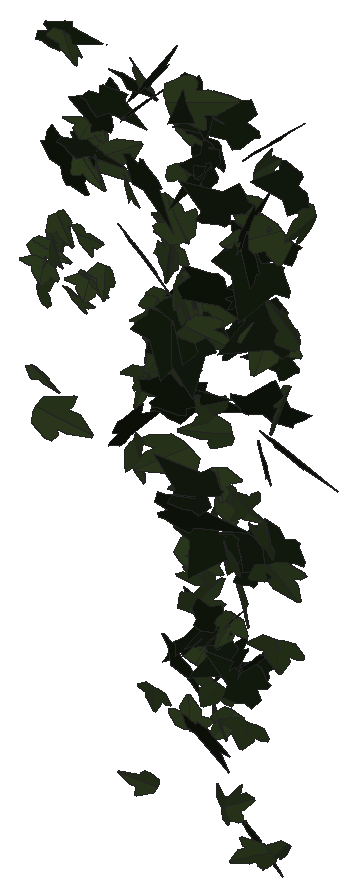
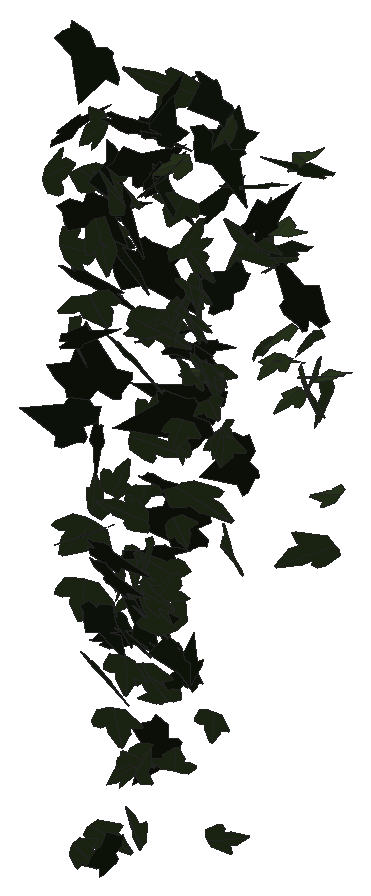
# SketchUp Ruby script. Lengths in inches.
U = 1.inch
M = Sketchup.active_model
def pt(a) = Geom::Point3d.new(a.map { |v| v * U })
def face(e, loops, mat)
  f = e.add_face(loops[0].map { |a| pt(a) })
  loops[1..].each { |l| e.add_face(l.map { |a| pt(a) }).erase! }
  f.material = f.back_material = mat if mat
  f
end
# faces: each face lists its corners as indices into pts; further lists are holes
def faces(e, pts, list, mat = nil) = list.each { |f| face(e, (f[0].is_a?(Array) ? f : [f]).map { |l| l.map { |i| pts[i] } }, mat) }
# xy, xz, yz: faces in a plane at the given z, y or x. An outline is a flat list of corners, or four numbers for a rectangle; further outlines are holes
def ring(l) = l.size == 4 ? [[l[0], l[1]], [l[2], l[1]], [l[2], l[3]], [l[0], l[3]]] : l.each_slice(2).to_a
def flat(e, list, mat, &to3) = list.each { |f| face(e, (f[0].is_a?(Array) ? f : [f]).map { |l| ring(l).map { |u, v| to3.(u, v) } }, mat) }
def xy(e, z, list, mat = nil) = flat(e, list, mat) { |x, y| [x, y, z] }
def xz(e, y, list, mat = nil) = flat(e, list, mat) { |x, z| [x, y, z] }
def yz(e, x, list, mat = nil) = flat(e, list, mat) { |y, z| [x, y, z] }
def lines(e, pts, list) = list.each { |a, b| e.add_line(pt(pts[a]), pt(pts[b])) }
# prism: a flat outline (further loops are holes) pulled along v
def prism(e, loops, v, mat = nil)
  f = face(e, loops, mat); d = Geom::Vector3d.new(v.map { |x| x * U })
  f.pushpull(f.normal.samedirection?(d) ? d.length : -d.length)
end
def box(e, o, s, mat = nil) = prism(e, [[o, [o[0] + s[0], o[1], o[2]], [o[0] + s[0], o[1] + s[1], o[2]], [o[0], o[1] + s[1], o[2]]]], [0, 0, s[2]], mat)
def at(x, y, z, deg = 0) = Geom::Transformation.translation(pt([x, y, z])) * Geom::Transformation.rotation(ORIGIN, Z_AXIS, deg.degrees)
def axes(o, x, y, z) = Geom::Transformation.new([*x, 0, *y, 0, *z, 0, *pt(o).to_a, 1])
def part(name) = M.definitions.add(name)
# library, detail: a bought-in or finely detailed component or shape, given as its bounding box
def library(name, o, s) = part(name).tap { |d| box(d.entities, o, s) }
def detail(e, o, s) = box(e.add_group.entities, o, s)
def put(e, d, t, mat = nil) = e.add_instance(d, t).tap { |i| i.material = mat if mat }
def group(e, t, mat = nil) = e.add_group.tap { |g| g.transformation = t; g.material = mat if mat }.entities
root = M.entities
M.materials.add("1026 AP 7946 SUNNY SIDE UP").color = [254, 231, 186]
M.materials.add("efeu1").color = [18, 25, 13]
M.materials.add("efeu2").color = [43, 57, 29]
c1 = part("ivyleaf_10")
p = [[0,0.5,-0.03],[-0.0625,2.02,-0.43],[-0.19,2.01,-0.46],[-0.54,1.05,-0.29],[-0.52,0.625,-0.18],[-0.83,0.76,-0.28],
  [-1.16,0.64,-0.33],[-1.15,0.33,-0.24],[-0.77,-0.39,0.02],[-0.3,-0.51,0.16],[0.04,-0.48,0.23],[-0.02,2.01,-0.4375],
  [-0.06,2.01,-0.43],[0.04,-0.49,0.23],[0.67,-0.49,0.14],[1.38,0.36,-0.2],[1.375,0.51,-0.24],[0.81,0.65,-0.19],
  [0.62,0.59,-0.15],[0.6,1.09,-0.28],[0.5,1.23,-0.31]]
faces(c1.entities,p,[[0,1,2,3,4,5,6,7,8,9,10],[11,12,0,13,14,15,16,17,18,19,20]],"efeu2")
c2 = part("ivyleaf_9")
p = [[1.54,2.16,1.25],[1.36,2.04,1.19],[-0.21,0.99,0.68],[-0.71,1.11,0.82],[-0.85,0.86,0.67],[-0.8,0.17,0.21],
  [-0.9,-0.01,0.1],[-0.67,-0.16,-0.02],[-0.08,-0.08,-0.05],[-0.03,-0.6,-0.4],[0.65,-0.88,-0.66],[0.83,-0.6,-0.49],
  [1.29,-0.42,-0.43],[1.8125,-0.07,-0.26],[1.21,0.44,0.15]]
faces(c2.entities,p,[[0,1,2,3,4,5,6,7,8,9,10,11,12,13,14]],"efeu1")
put(root,c1,axes([138.98,210.22,263.24],[-0.26832,-0.09266,0.10652],[0.15209,-0.19714,-0.01861],[0.15749,0.03251,0.19947]),"1026 AP 7946 SUNNY SIDE UP")
put(root,c1,axes([141.6,210.05,255.69],[-0.31273,0.03362,0.02954],[-0.04908,-0.01456,-0.20692],[-0.0489,-0.20039,0.01878]),"1026 AP 7946 SUNNY SIDE UP")
put(root,c2,axes([143.76,210.15,256.46],[-0.25605,-0.21365,-0.05442],[-0.05292,-0.03924,0.27649],[-0.34152,0.16625,-0.00204]),"1026 AP 7946 SUNNY SIDE UP")
put(root,c2,axes([142,210.32,256.35],[0.31816,-0.22092,-0.16843],[0.20052,-0.10262,0.30721],[-0.3815,-0.23818,0.02101]),"1026 AP 7946 SUNNY SIDE UP")
put(root,c2,axes([143.74,210.33,264.84],[-0.29155,-0.31885,0.04974],[0.01185,-0.06203,-0.37839],[0.50737,-0.18177,0.03742]),"1026 AP 7946 SUNNY SIDE UP")
put(root,c2,axes([141.14,210.23,265.92],[0.26357,-0.32189,0.03584],[0.00376,-0.03999,-0.37373],[0.50938,0.16685,-0.01578]),"1026 AP 7946 SUNNY SIDE UP")
put(root,c1,axes([139.97,210.27,263.22],[-0.30788,-0.07706,0.05458],[0.11552,-0.20293,-0.02532],[0.0916,-0.00305,0.2154]),"1026 AP 7946 SUNNY SIDE UP")
put(root,c1,axes([143.17,210.25,257.56],[0.14453,0.17083,-0.16949],[-0.10294,-0.1524,-0.20041],[-0.35954,0.1123,-0.01076]),"1026 AP 7946 SUNNY SIDE UP")
put(root,c2,axes([142.03,210.28,262.86],[-0.30127,-0.16523,-0.24528],[0.39598,0.04422,-0.24108],[0.22307,-0.30166,0.09668]),"1026 AP 7946 SUNNY SIDE UP")
put(root,c2,axes([143.08,210.27,265.71],[0.06562,0.03036,0.30626],[-0.45026,-0.08115,0.0495],[0.1334,-0.28884,0.01644]),"1026 AP 7946 SUNNY SIDE UP")
put(root,c1,axes([142.92,210.16,256.16],[-0.34394,-0.02236,0.12398],[-0.18185,-0.04373,-0.22494],[0.06363,-0.24586,0.02724]),"1026 AP 7946 SUNNY SIDE UP")
put(root,c2,axes([141.7,210.07,261.63],[0.17769,0.01894,0.30716],[0.4696,-0.00543,-0.11633],[-0.00256,0.31871,-0.01836]),"1026 AP 7946 SUNNY SIDE UP")
put(root,c2,axes([140.98,209.88,260.74],[0.12516,0.14997,0.31618],[0.26676,0.25516,-0.17277],[-0.46482,0.18682,-0.01401]),"1026 AP 7946 SUNNY SIDE UP")
put(root,c2,axes([143.1875,210.25,256.81],[-0.40171,0.02984,0.02023],[-0.03496,-0.02339,-0.26379],[-0.04378,-0.25515,0.02502]),"1026 AP 7946 SUNNY SIDE UP")
put(root,c1,axes([143.41,209.97,254.0625],[-0.00784,0.02709,0.27849],[-0.07168,0.26631,-0.02682],[-0.4209,-0.04585,-0.00062]),"1026 AP 7946 SUNNY SIDE UP")
put(root,c2,axes([140.92,210.36,264.24],[0.23132,-0.24892,0.20326],[0.14646,-0.1757,-0.29879],[0.47893,0.17395,-0.0068]),"1026 AP 7946 SUNNY SIDE UP")
put(root,c2,axes([141.78,210.35,262.9],[-0.2621,-0.26595,-0.02368],[0.04161,0.00871,-0.32278],[0.41747,-0.16784,0.01731]),"1026 AP 7946 SUNNY SIDE UP")
put(root,c2,axes([143.38,210.27,257.04],[-0.29867,0.12568,-0.13501],[0.15186,-0.09188,-0.23425],[-0.24272,-0.21213,0.01957]),"1026 AP 7946 SUNNY SIDE UP")
put(root,c1,axes([138.79,210.25,261.03],[0.00803,-0.18886,0.07584],[0.30325,-0.0189,-0.06294],[0.10008,0.07244,0.18463]),"1026 AP 7946 SUNNY SIDE UP")
put(root,c2,axes([142.97,210.25,257.34],[-0.35126,0.10724,-0.02573],[0.02114,-0.03088,-0.25446],[-0.17206,-0.22272,0.02126]),"1026 AP 7946 SUNNY SIDE UP")
put(root,c1,axes([140.24,210.36,263.46],[-0.10201,-0.17563,0.12827],[0.1628,-0.14031,-0.14796],[0.29784,0.01654,0.12481]),"1026 AP 7946 SUNNY SIDE UP")
put(root,c2,axes([143.01,210.24,264.17],[0.03459,0.13881,-0.34969],[-0.43407,-0.21872,-0.1116],[-0.38135,0.26154,0.0953]),"1026 AP 7946 SUNNY SIDE UP")
put(root,c2,axes([144.2,209.96,267.58],[0.12837,0.33147,0.16836],[0.02917,0.16155,-0.35021],[-0.57907,0.08162,0.01968]),"1026 AP 7946 SUNNY SIDE UP")
put(root,c2,axes([142.58,210.24,259.89],[-0.38041,-0.09691,-0.142],[-0.21271,-0.03045,0.26755],[-0.15676,0.27649,-0.01847]),"1026 AP 7946 SUNNY SIDE UP")
put(root,c2,axes([143.59,210.14,265.2],[0.09755,-0.04066,-0.38485],[-0.58547,0.04263,-0.06827],[0.07692,0.37605,-0.03162]),"1026 AP 7946 SUNNY SIDE UP")
put(root,c1,axes([141.28,210.32,253.6],[-0.08349,-0.02972,-0.20093],[-0.29572,-0.05283,0.06078],[-0.09287,0.19494,-0.01291]),"1026 AP 7946 SUNNY SIDE UP")
put(root,c1,axes([141.64,210.3,262.55],[0.40251,-0.21261,-0.06265],[-0.09805,0.01793,-0.34168],[0.33307,0.26222,-0.02488]),"1026 AP 7946 SUNNY SIDE UP")
put(root,c2,axes([142.72,210.22,257.01],[0.09106,0.26368,0.08717],[-0.04006,-0.07947,0.27754],[0.43287,-0.06282,0.00735]),"1026 AP 7946 SUNNY SIDE UP")
put(root,c1,axes([141.12,210.36,261.54],[0.07408,0.15737,-0.12689],[-0.05346,-0.11932,-0.16992],[-0.31053,0.05809,-0.00102]),"1026 AP 7946 SUNNY SIDE UP")
put(root,c2,axes([141.85,210.21,259.33],[0.33666,0.01357,0.26927],[0.41,-0.03918,-0.21823],[0.03426,0.33554,-0.03438]),"1026 AP 7946 SUNNY SIDE UP")
put(root,c1,axes([142.09,210.1875,267.62],[0.16546,-0.01515,-0.3647],[0.54382,0.08429,0.10271],[0.12054,-0.35949,0.03723]),"1026 AP 7946 SUNNY SIDE UP")
put(root,c1,axes([144.16,210.3,257.4],[-0.42519,-0.08595,0.00603],[0.00354,-0.02791,-0.29112],[0.13547,-0.26904,0.02653]),"1026 AP 7946 SUNNY SIDE UP")
put(root,c2,axes([143.83,210.27,257.08],[-0.10898,0.24451,-0.10809],[0.03027,-0.10497,-0.26226],[-0.41815,-0.07132,0.00919]),"1026 AP 7946 SUNNY SIDE UP")
put(root,c2,axes([142.18,210.625,267.55],[0.11944,-0.19514,-0.32586],[0.2779,-0.26377,0.21056],[-0.51241,-0.18854,0.03824]),"1026 AP 7946 SUNNY SIDE UP")
put(root,c2,axes([142.77,210.25,257.32],[0.00556,0.01588,0.24924],[-0.23403,0.19104,-0.00957],[-0.30078,-0.14835,0.01205]),"1026 AP 7946 SUNNY SIDE UP")
put(root,c2,axes([143.69,210.23,264.46],[-0.26245,0.33183,0.04085],[-0.05802,0.02364,-0.38183],[-0.52192,-0.16949,0.0219]),"1026 AP 7946 SUNNY SIDE UP")
put(root,c1,axes([142.35,210.25,263.12],[-0.19503,-0.11717,-0.26327],[0.37231,0.10573,-0.16815],[0.23656,-0.26301,0.04759]),"1026 AP 7946 SUNNY SIDE UP")
put(root,c1,axes([144.15,210.5,262.31],[0.24325,-0.26209,0.15842],[0.09853,-0.14304,-0.31389],[0.46876,0.16607,-0.01623]),"1026 AP 7946 SUNNY SIDE UP")
put(root,c1,axes([143.86,210.4375,265.48],[0.36569,-0.01285,-0.27554],[-0.41891,-0.04583,-0.23671],[-0.04126,0.35141,-0.03886]),"1026 AP 7946 SUNNY SIDE UP")
put(root,c1,axes([144.52,210.2,263.79],[-0.15496,0.08193,-0.33439],[-0.35451,0.23452,0.13269],[0.39006,0.2457,-0.01225]),"1026 AP 7946 SUNNY SIDE UP")
put(root,c2,axes([142.38,210.3,255.12],[0.47628,-0.05284,-0.11752],[-0.18146,-0.00076,-0.31614],[0.07735,0.32356,-0.01799]),"1026 AP 7946 SUNNY SIDE UP")
put(root,c1,axes([140.25,210.16,265.85],[-0.11224,0.14454,0.33301],[-0.34995,0.2371,-0.15887],[-0.43154,-0.22987,0.04222]),"1026 AP 7946 SUNNY SIDE UP")
put(root,c2,axes([142.15,210.14,256.68],[-0.24883,0.26623,-0.12954],[-0.07862,0.11812,0.31933],[0.45728,0.16518,-0.01559]),"1026 AP 7946 SUNNY SIDE UP")
put(root,c1,axes([142.35,210.42,258.04],[-0.31287,-0.0309,-0.0969],[-0.14863,-0.0022,0.20711],[-0.04543,0.22,-0.01023]),"1026 AP 7946 SUNNY SIDE UP")
put(root,c1,axes([143.21,210.47,258.02],[-0.15256,0.18734,-0.16128],[0.09342,-0.14646,-0.21786],[-0.37345,-0.11317,0.01139]),"1026 AP 7946 SUNNY SIDE UP")
put(root,c1,axes([143.67,210.48,252.98],[-0.18074,-0.05757,0.20926],[-0.25211,-0.12724,-0.13115],[0.21674,-0.196,0.02195]),"1026 AP 7946 SUNNY SIDE UP")
put(root,c1,axes([143.29,210.55,259.75],[-0.09862,-0.17926,-0.17408],[-0.11595,-0.15162,0.19418],[-0.36845,0.09569,-0.01451]),"1026 AP 7946 SUNNY SIDE UP")
put(root,c2,axes([141.34,210.14,267.6875],[-0.2364,0.24822,-0.21717],[-0.16616,0.18408,0.30001],[0.48587,0.18372,-0.00307]),"1026 AP 7946 SUNNY SIDE UP")
put(root,c2,axes([140.8,210.61,267.3],[-0.2359,-0.11468,0.15811],[0.13556,-0.21495,-0.07957],[0.26996,0.00773,0.17812]),"1026 AP 7946 SUNNY SIDE UP")
put(root,c1,axes([142.48,210.58,261.36],[-0.13794,-0.19271,-0.18575],[-0.13792,-0.15669,0.2169],[-0.39013,0.12353,-0.011]),"1026 AP 7946 SUNNY SIDE UP")
put(root,c2,axes([142.09,210.68,263.15],[-0.24608,-0.30492,0.08143],[0.05383,-0.10606,-0.34473],[0.49307,-0.1406,0.07828]),"1026 AP 7946 SUNNY SIDE UP")
put(root,c1,axes([139.98,210.3,263.24],[0.29665,-0.083,-0.0796],[0.09356,0.1999,-0.0708],[0.15119,0.03915,0.19999]),"1026 AP 7946 SUNNY SIDE UP")
put(root,c1,axes([139.01,210.18,262.87],[-0.03711,0.08734,0.35736],[-0.24993,0.30832,-0.08944],[-0.50304,-0.15963,0.01807]),"1026 AP 7946 SUNNY SIDE UP")
put(root,c2,axes([143.51,210.15,265.4],[0.04458,0.06281,0.38591],[0.2062,0.35055,-0.06879],[-0.55993,0.13409,0.00539]),"1026 AP 7946 SUNNY SIDE UP")
put(root,c1,axes([142.03,210.35,263.5],[-0.02137,0.2768,0.09716],[-0.0234,0.09206,-0.28478],[-0.45842,-0.0176,0.01001]),"1026 AP 7946 SUNNY SIDE UP")
put(root,c1,axes([143.75,210.47,259.18],[-0.3468,0.14663,0.0547],[0.08747,-0.01042,0.27187],[0.2286,0.22642,-0.02103]),"1026 AP 7946 SUNNY SIDE UP")
put(root,c1,axes([139.54,210.35,262.76],[0.26003,-0.13196,-0.05972],[0.15404,0.16718,-0.10453],[0.16558,0.0517,0.19102]),"1026 AP 7946 SUNNY SIDE UP")
put(root,c1,axes([138.7,210.47,263.43],[0.00846,-0.21219,-0.05812],[0.33604,0.01742,-0.04741],[0.07705,-0.05267,0.21314]),"1026 AP 7946 SUNNY SIDE UP")
put(root,c1,axes([139.01,210.45,263.52],[0.12536,-0.20853,-0.03803],[0.13076,0.066,-0.20525],[0.30589,0.05725,0.10333]),"1026 AP 7946 SUNNY SIDE UP")
put(root,c2,axes([143.96,210.6,263.61],[-0.5613,0.01436,0.02484],[-0.04019,-0.04181,-0.36565],[-0.01796,-0.35533,0.04192]),"1026 AP 7946 SUNNY SIDE UP")
put(root,c1,axes([139.1,210.5,264.07],[-0.02988,-0.23556,-0.00941],[0.21592,-0.00471,-0.19827],[0.30119,-0.02,0.14121]),"1026 AP 7946 SUNNY SIDE UP")
put(root,c2,axes([142.51,210.68,258.85],[-0.331,-0.2246,0.04157],[-0.02208,-0.04377,-0.31674],[0.3585,-0.21007,0.01887]),"1026 AP 7946 SUNNY SIDE UP")
put(root,c1,axes([142.24,210.41,257.48],[-0.16605,-0.25432,0.16543],[0.07701,0.15493,0.28431],[-0.46785,0.11577,-0.01192]),"1026 AP 7946 SUNNY SIDE UP")
put(root,c1,axes([141.8,210.51,264.78],[0.08902,0.33263,0.0434],[-0.02434,-0.03817,0.34726],[0.52628,-0.05803,0.00872]),"1026 AP 7946 SUNNY SIDE UP")
put(root,c1,axes([140.625,210.5,265.3125],[0.18434,-0.20402,-0.02188],[0.1573,0.07713,-0.20512],[0.28138,0.09055,0.129]),"1026 AP 7946 SUNNY SIDE UP")
put(root,c1,axes([139.625,210.58,265.37],[-0.07078,-0.23207,0.0041],[0.28633,-0.03865,-0.15044],[0.22638,-0.02368,0.19156]),"1026 AP 7946 SUNNY SIDE UP")
put(root,c1,axes([142.21,210.38,258.39],[0.27911,0.09157,-0.23935],[0.2994,0.13579,0.20534],[0.25525,-0.25941,0.02087]),"1026 AP 7946 SUNNY SIDE UP")
put(root,c1,axes([141.65,210.63,260.26],[0.37779,0.03426,-0.24996],[-0.36225,-0.08498,-0.24768],[-0.13217,0.33086,-0.03565]),"1026 AP 7946 SUNNY SIDE UP")
put(root,c1,axes([141.91,210.53,263.73],[-0.00079,0.35802,-0.04178],[0.00239,-0.04258,-0.36908],[-0.56692,-0.00068,-0.0015]),"1026 AP 7946 SUNNY SIDE UP")
put(root,c1,axes([143.29,210.55,255.35],[-0.36654,-0.06918,0.06119],[-0.07864,-0.04059,-0.24951],[0.12036,-0.2372,0.02331]),"1026 AP 7946 SUNNY SIDE UP")
put(root,c1,axes([141.62,210.31,264.09],[0.00876,0.09908,-0.31032],[-0.04509,0.30076,0.10294],[0.49741,0.02552,0.0148]),"1026 AP 7946 SUNNY SIDE UP")
put(root,c1,axes([143.92,210.51,258.72],[-0.40507,-0.09272,-0.13679],[0.2073,0.02312,-0.28112],[0.14672,-0.28865,0.01955]),"1026 AP 7946 SUNNY SIDE UP")
put(root,c1,axes([139.67,210.42,263.97],[0.23213,-0.13804,-0.12059],[0.16067,0.18774,-0.09487],[0.23393,0.00803,0.18482]),"1026 AP 7946 SUNNY SIDE UP")
put(root,c1,axes([139.6,210.73,266.01],[-0.34515,-0.0403,0.07754],[0.09641,-0.21905,0.0619],[0.09387,0.07679,0.22151]),"1026 AP 7946 SUNNY SIDE UP")
put(root,c1,axes([141.93,210.56,263.64],[0.10517,0.35126,-0.03112],[0.0016,-0.03297,-0.36848],[-0.55463,0.06651,-0.00696]),"1026 AP 7946 SUNNY SIDE UP")
put(root,c1,axes([139.0625,210.73,267.57],[-0.17358,-0.1635,0.16121],[0.2943,-0.16459,-0.04186],[0.20186,0.09938,0.19966]),"1026 AP 7946 SUNNY SIDE UP")
put(root,c2,axes([141.83,210.35,261.53],[0.06196,0.10801,-0.34122],[0.1242,0.32251,0.11969],[0.53448,-0.08747,0.01174]),"1026 AP 7946 SUNNY SIDE UP")
put(root,c1,axes([143.67,210.67,263.26],[0.36855,0.22807,-0.12893],[-0.10451,-0.11215,-0.33598],[-0.39651,0.24155,-0.03128]),"1026 AP 7946 SUNNY SIDE UP")
put(root,c2,axes([144.16,210.82,266.37],[0.02617,-0.25139,-0.18066],[0.07928,-0.16955,0.25642],[-0.47409,-0.04223,0.03291]),"1026 AP 7946 SUNNY SIDE UP")
put(root,c1,axes([142.59,210.6875,260.94],[-0.07947,0.00086,0.27651],[-0.34125,-0.16083,-0.04251],[0.24833,-0.22074,0.03008]),"1026 AP 7946 SUNNY SIDE UP")
put(root,c1,axes([141.09,210.625,262.76],[-0.18503,-0.17704,0.01007],[0.00524,-0.01514,-0.21879],[0.27885,-0.11719,0.01079]),"1026 AP 7946 SUNNY SIDE UP")
put(root,c1,axes([143.05,210.59,256.45],[-0.38509,0.05392,0.04721],[-0.07949,-0.01937,-0.25669],[-0.07741,-0.24835,0.02874]),"1026 AP 7946 SUNNY SIDE UP")
put(root,c2,axes([141.13,210.53,267.19],[-0.14276,0.34778,-0.0675],[0.01382,-0.06744,-0.37058],[-0.55688,-0.09083,0.0081]),"1026 AP 7946 SUNNY SIDE UP")
put(root,c1,axes([143.07,210.79,265.49],[-0.0192,-0.05071,-0.32168],[0.3316,-0.23384,0.02929],[-0.37016,-0.20685,0.04292]),"1026 AP 7946 SUNNY SIDE UP")
put(root,c1,axes([141.83,210.69,259.61],[-0.11105,-0.18118,0.05687],[-0.02364,-0.05446,-0.20057],[0.29736,-0.072,0.00529]),"1026 AP 7946 SUNNY SIDE UP")
put(root,c1,axes([141.16,210.56,262.72],[0.2162,-0.16208,0.00759],[0.25518,0.13722,-0.00826],[0.00214,0.01201,0.21885]),"1026 AP 7946 SUNNY SIDE UP")
put(root,c2,axes([142.25,210.86,266.03],[-0.06193,-0.03132,0.29302],[-0.24024,-0.24068,-0.05047],[0.38077,-0.15694,0.01581]),"1026 AP 7946 SUNNY SIDE UP")
put(root,c1,axes([140.75,210.6,267.6],[0.21055,-0.20509,-0.02441],[0.19463,0.10134,-0.19188],[0.25956,0.09037,0.16369]),"1026 AP 7946 SUNNY SIDE UP")
put(root,c2,axes([143.53,210.71,261.66],[0.51075,0.05213,0.11446],[-0.18076,0.02158,0.33683],[0.06635,-0.34252,0.03658]),"1026 AP 7946 SUNNY SIDE UP")
put(root,c2,axes([139.37,210.64,265.6875],[0.23197,-0.19483,-0.03158],[0.18983,0.11853,-0.18352],[0.2449,0.09267,0.17216]),"1026 AP 7946 SUNNY SIDE UP")
put(root,c2,axes([142.14,210.75,266.1],[-0.36059,0.15533,-0.19461],[0.21979,-0.13072,-0.28498],[-0.31687,-0.26743,0.02379]),"1026 AP 7946 SUNNY SIDE UP")
put(root,c2,axes([143.74,210.75,265.1],[0.04394,0.12179,-0.26439],[-0.09405,-0.25029,-0.13019],[-0.43768,0.06601,0.00143]),"1026 AP 7946 SUNNY SIDE UP")
put(root,c1,axes([142.83,210.59,258.63],[-0.29398,0.15481,0.11289],[-0.15594,0.04993,-0.24869],[-0.25329,-0.21042,0.02208]),"1026 AP 7946 SUNNY SIDE UP")
put(root,c2,axes([139.92,210.68,266.76],[0.16195,-0.2055,-0.08572],[0.17013,0.12571,-0.18373],[0.3035,0.03919,0.14873]),"1026 AP 7946 SUNNY SIDE UP")
put(root,c1,axes([141.91,210.65,254.91],[0.31852,0.10539,-0.00287],[-0.00957,0.01901,0.23447],[0.16552,-0.2017,0.01909]),"1026 AP 7946 SUNNY SIDE UP")
put(root,c1,axes([141.8,210.69,263.63],[-0.28025,0.2986,-0.06599],[0.02581,-0.06666,-0.35806],[-0.48008,-0.1779,0.01927]),"1026 AP 7946 SUNNY SIDE UP")
put(root,c1,axes([138.86,210.51,260.1],[0.11762,0.16921,0.29681],[0.23393,0.24639,-0.18806],[-0.46897,0.16535,-0.01937]),"1026 AP 7946 SUNNY SIDE UP")
put(root,c1,axes([141.5,210.61,264.79],[0.10612,-0.03381,-0.21992],[-0.23465,0.15422,-0.07292],[0.24544,0.16206,0.02537]),"1026 AP 7946 SUNNY SIDE UP")
put(root,c1,axes([140.82,210.72,261.54],[-0.25515,-0.12333,-0.00555],[0.03032,-0.01769,-0.2084],[0.19169,-0.16137,0.02558]),"1026 AP 7946 SUNNY SIDE UP")
put(root,c1,axes([142.5,210.71,260.05],[0.20936,0.17747,0.01097],[0.02424,0.00047,-0.22823],[-0.27842,0.1335,-0.01162]),"1026 AP 7946 SUNNY SIDE UP")
put(root,c2,axes([142.11,210.875,267.07],[-0.29936,-0.0494,0.14633],[0.11351,-0.23123,0.01545],[0.20792,0.05511,0.20225]),"1026 AP 7946 SUNNY SIDE UP")
put(root,c1,axes([142.52,210.8125,253.38],[-0.17681,0.08868,0.22294],[0.30812,-0.09433,0.1445],[0.19938,0.22441,-0.02561]),"1026 AP 7946 SUNNY SIDE UP")
put(root,c1,axes([141.6,210.86,261.25],[0.03705,-0.1414,0.15558],[0.09383,-0.14172,-0.14635],[0.31244,0.05932,0.0255]),"1026 AP 7946 SUNNY SIDE UP")
put(root,c1,axes([140.97,210.8,262.91],[0.27154,-0.12131,0.03589],[0.03625,-0.02891,-0.21733],[0.19542,0.17392,-0.00955]),"1026 AP 7946 SUNNY SIDE UP")
put(root,c1,axes([143.4,210.79,264.73],[-0.09334,-0.35859,0.00087],[0.01109,-0.00408,-0.37438],[0.56375,-0.05929,0.00751]),"1026 AP 7946 SUNNY SIDE UP")
put(root,c1,axes([142.59,210.77,259.51],[0.01057,0.00494,0.29795],[0.45077,0.03823,-0.00731],[-0.06028,0.28673,-0.00245]),"1026 AP 7946 SUNNY SIDE UP")
put(root,c1,axes([139.85,210.75,265.5],[0.33953,-0.06666,-0.256],[0.39581,-0.00996,0.22838],[-0.08083,-0.32877,0.04299]),"1026 AP 7946 SUNNY SIDE UP")
put(root,c2,axes([143.51,210.69,260.8],[0.19451,-0.07257,-0.22373],[-0.32278,0.07317,-0.1455],[0.15814,0.23861,-0.02177]),"1026 AP 7946 SUNNY SIDE UP")
put(root,c1,axes([143.58,210.56,266.57],[0.04262,0.01126,0.30383],[-0.12211,0.28594,-0.00222],[-0.44763,-0.07693,0.02954]),"1026 AP 7946 SUNNY SIDE UP")
put(root,c1,axes([144.23,211.04,265.61],[-0.00334,-0.02504,0.34224],[0.13632,-0.32096,-0.02622],[0.50604,0.0863,0.00932]),"1026 AP 7946 SUNNY SIDE UP")
put(root,c1,axes([141.37,210.77,264.22],[0.20784,-0.1674,-0.06577],[-0.0176,0.07032,-0.21662],[0.28063,0.12839,0.03513]),"1026 AP 7946 SUNNY SIDE UP")
put(root,c1,axes([141.6875,210.75,265.86],[0.30559,0.09597,0.08781],[0.06782,0.09588,-0.21332],[-0.1895,0.18908,0.06527]),"1026 AP 7946 SUNNY SIDE UP")
put(root,c1,axes([142.0625,210.73,256.22],[0.27985,0.098,-0.1068],[0.1256,0.06995,0.20867],[0.18662,-0.19403,0.01971]),"1026 AP 7946 SUNNY SIDE UP")
put(root,c2,axes([143.72,210.9,260.9375],[0.30524,-0.20297,0.19195],[0.26097,-0.09753,-0.28638],[0.34735,0.25163,0.04648]),"1026 AP 7946 SUNNY SIDE UP")
put(root,c1,axes([141.64,210.76,266.63],[0.21682,-0.19185,0.02056],[0.28741,0.1215,-0.09195],[0.09744,0.06851,0.22547]),"1026 AP 7946 SUNNY SIDE UP")
put(root,c1,axes([140.88,210.78,261.68],[-0.07685,0.19545,0.03974],[-0.04947,0.03051,-0.20605],[-0.30899,-0.0535,0.0231]),"1026 AP 7946 SUNNY SIDE UP")
put(root,c1,axes([140.98,210.88,262.32],[0.10199,0.18071,-0.08412],[-0.08767,-0.06693,-0.19616],[-0.29993,0.08102,0.02873]),"1026 AP 7946 SUNNY SIDE UP")
put(root,c2,axes([139.79,211.07,266.16],[-0.00908,0.0294,0.36168],[-0.35862,-0.26772,0.01768],[0.42189,-0.22694,0.02281]),"1026 AP 7946 SUNNY SIDE UP")
put(root,c2,axes([138.79,211,264.82],[-0.06508,0.03556,0.3884],[0.28088,-0.33235,0.05058],[0.52469,0.18233,0.0211]),"1026 AP 7946 SUNNY SIDE UP")
put(root,c1,axes([140.37,211.02,259.7],[0.18749,-0.05011,0.29988],[0.37212,-0.17214,-0.13128],[0.27865,0.2636,-0.02646]),"1026 AP 7946 SUNNY SIDE UP")
put(root,c1,axes([142.43,210.85,263.36],[0.14427,-0.02119,-0.32046],[-0.4782,0.06479,-0.09662],[0.10715,0.31766,0.00027]),"1026 AP 7946 SUNNY SIDE UP")
put(root,c1,axes([141.08,210.91,263.04],[0.31056,-0.08059,0.01369],[0.01036,-0.02014,-0.21925],[0.12814,0.19696,-0.01546]),"1026 AP 7946 SUNNY SIDE UP")
put(root,c1,axes([142.55,210.99,255.08],[0.1771,0.14211,-0.18578],[-0.15212,-0.15377,-0.18716],[-0.32851,0.14782,-0.01349]),"1026 AP 7946 SUNNY SIDE UP")
put(root,c2,axes([142.86,210.98,267.11],[-0.44405,0.0353,0.15888],[-0.24772,-0.03847,-0.28872],[-0.01925,-0.31937,0.05042]),"1026 AP 7946 SUNNY SIDE UP")
put(root,c1,axes([143.68,211,252.86],[-0.04755,-0.17408,0.14253],[-0.02846,-0.13824,-0.18277],[0.34945,-0.03494,0.00451]),"1026 AP 7946 SUNNY SIDE UP")
put(root,c1,axes([141.29,210.97,262.8],[0.25504,-0.0475,0.13398],[0.19112,-0.04794,-0.17413],[0.10508,0.20247,-0.00848]),"1026 AP 7946 SUNNY SIDE UP")
put(root,c2,axes([138.65,210.86,267.53],[0.27714,-0.16748,-0.02725],[0.22752,0.16796,-0.10515],[0.13853,0.05918,0.22722]),"1026 AP 7946 SUNNY SIDE UP")
put(root,c1,axes([141.28,210.96,264.4375],[0.33795,-0.05167,0.0359],[0.04648,-0.02683,-0.22704],[0.08657,0.21612,-0.01824]),"1026 AP 7946 SUNNY SIDE UP")
put(root,c1,axes([138.74,211.06,263.48],[0.34949,-0.22272,0.15118],[0.13421,-0.12331,-0.32392],[0.39849,0.23686,-0.0235]),"1026 AP 7946 SUNNY SIDE UP")
put(root,c2,axes([141.88,211.19,266.35],[-0.07679,-0.25738,0.22567],[-0.04004,-0.21938,-0.27088],[0.53143,-0.05372,0.0122]),"1026 AP 7946 SUNNY SIDE UP")
put(root,c2,axes([143.6,211.14,258.94],[-0.18902,-0.24958,0.11076],[0.0163,-0.12318,-0.27968],[0.42788,-0.10556,0.05958]),"1026 AP 7946 SUNNY SIDE UP")
put(root,c2,axes([142.97,210.98,253.02],[0.29503,-0.20044,0.02726],[0.01169,-0.03079,-0.28258],[0.31793,0.18714,-0.01491]),"1026 AP 7946 SUNNY SIDE UP")
put(root,c1,axes([141.24,210.89,264.53],[-0.25003,0.15363,0.03922],[-0.08444,-0.00288,-0.22425],[-0.23376,-0.16328,0.03906]),"1026 AP 7946 SUNNY SIDE UP")
put(root,c2,axes([143.47,210.85,256.4],[-0.21305,0.18365,0.09899],[-0.10084,0.07071,-0.23452],[-0.30913,-0.14964,0.00828]),"1026 AP 7946 SUNNY SIDE UP")
put(root,c1,axes([142.28,210.88,258.15],[0.06689,0.01151,0.22948],[-0.34573,0.0399,0.04138],[-0.05836,-0.22318,0.01788]),"1026 AP 7946 SUNNY SIDE UP")
put(root,c2,axes([143.79,211.11,262.63],[-0.17319,-0.04445,0.23617],[-0.28338,-0.14543,-0.11898],[0.2341,-0.20893,0.0307]),"1026 AP 7946 SUNNY SIDE UP")
put(root,c2,axes([143.3,210.95,258.71],[-0.18686,-0.0735,-0.23946],[-0.35165,-0.0689,0.14008],[-0.15099,0.25142,-0.02991]),"1026 AP 7946 SUNNY SIDE UP")
put(root,c1,axes([141.2,211.02,263.82],[0.26315,-0.12814,0.06001],[0.06371,-0.04399,-0.21716],[0.21245,0.1719,-0.00921]),"1026 AP 7946 SUNNY SIDE UP")
put(root,c1,axes([142.29,210.82,259.05],[-0.02111,0.05457,0.21108],[-0.17164,0.17386,-0.05414],[-0.28527,-0.10865,0.01695]),"1026 AP 7946 SUNNY SIDE UP")
put(root,c1,axes([141.55,210.93,261.7],[-0.19155,-0.15423,-0.08028],[0.08678,0.05449,-0.20195],[0.25683,-0.13345,0.00836]),"1026 AP 7946 SUNNY SIDE UP")
put(root,c1,axes([142.41,210.93,254.79],[-0.24266,0.18165,-0.08468],[-0.073,0.06969,0.24578],[0.30559,0.1609,-0.00854]),"1026 AP 7946 SUNNY SIDE UP")
put(root,c2,axes([143.17,210.89,258.23],[-0.12559,0.10771,0.22549],[-0.24338,0.15481,-0.13615],[-0.29536,-0.17336,0.01631]),"1026 AP 7946 SUNNY SIDE UP")
put(root,c1,axes([141.23,211.04,263.93],[0.3327,-0.05662,0.01532],[0.01425,-0.02464,-0.22471],[0.09107,0.2107,-0.02082]),"1026 AP 7946 SUNNY SIDE UP")
put(root,c2,axes([142.8125,210.93,262.75],[-0.26133,0.19983,0.08531],[-0.10559,0.0501,-0.26677],[-0.3226,-0.17827,0.01821]),"1026 AP 7946 SUNNY SIDE UP")
